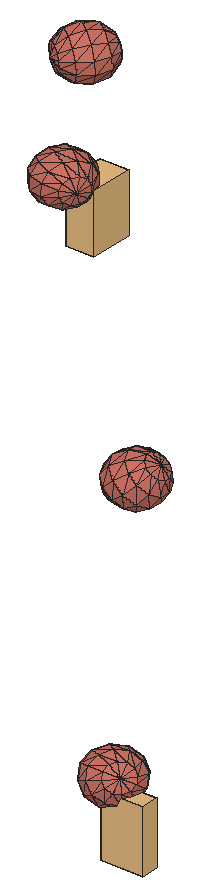
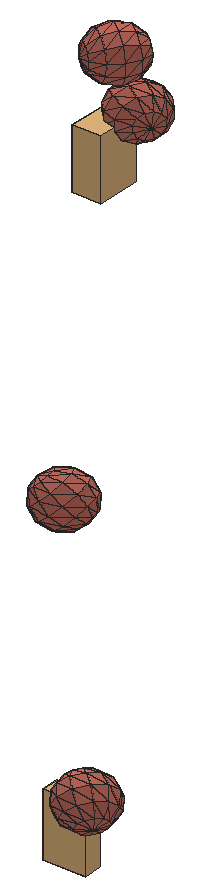
# SketchUp Ruby script. Lengths in inches.
U = 1.inch
M = Sketchup.active_model
def pt(a) = Geom::Point3d.new(a.map { |v| v * U })
def face(e, loops, mat)
  f = e.add_face(loops[0].map { |a| pt(a) })
  loops[1..].each { |l| e.add_face(l.map { |a| pt(a) }).erase! }
  f.material = f.back_material = mat if mat
  f
end
# faces: each face lists its corners as indices into pts; further lists are holes
def faces(e, pts, list, mat = nil) = list.each { |f| face(e, (f[0].is_a?(Array) ? f : [f]).map { |l| l.map { |i| pts[i] } }, mat) }
# xy, xz, yz: faces in a plane at the given z, y or x. An outline is a flat list of corners, or four numbers for a rectangle; further outlines are holes
def ring(l) = l.size == 4 ? [[l[0], l[1]], [l[2], l[1]], [l[2], l[3]], [l[0], l[3]]] : l.each_slice(2).to_a
def flat(e, list, mat, &to3) = list.each { |f| face(e, (f[0].is_a?(Array) ? f : [f]).map { |l| ring(l).map { |u, v| to3.(u, v) } }, mat) }
def xy(e, z, list, mat = nil) = flat(e, list, mat) { |x, y| [x, y, z] }
def xz(e, y, list, mat = nil) = flat(e, list, mat) { |x, z| [x, y, z] }
def yz(e, x, list, mat = nil) = flat(e, list, mat) { |y, z| [x, y, z] }
def lines(e, pts, list) = list.each { |a, b| e.add_line(pt(pts[a]), pt(pts[b])) }
# prism: a flat outline (further loops are holes) pulled along v
def prism(e, loops, v, mat = nil)
  f = face(e, loops, mat); d = Geom::Vector3d.new(v.map { |x| x * U })
  f.pushpull(f.normal.samedirection?(d) ? d.length : -d.length)
end
def box(e, o, s, mat = nil) = prism(e, [[o, [o[0] + s[0], o[1], o[2]], [o[0] + s[0], o[1] + s[1], o[2]], [o[0], o[1] + s[1], o[2]]]], [0, 0, s[2]], mat)
def at(x, y, z, deg = 0) = Geom::Transformation.translation(pt([x, y, z])) * Geom::Transformation.rotation(ORIGIN, Z_AXIS, deg.degrees)
def axes(o, x, y, z) = Geom::Transformation.new([*x, 0, *y, 0, *z, 0, *pt(o).to_a, 1])
def part(name) = M.definitions.add(name)
# library, detail: a bought-in or finely detailed component or shape, given as its bounding box
def library(name, o, s) = part(name).tap { |d| box(d.entities, o, s) }
def detail(e, o, s) = box(e.add_group.entities, o, s)
def put(e, d, t, mat = nil) = e.add_instance(d, t).tap { |i| i.material = mat if mat }
def group(e, t, mat = nil) = e.add_group.tap { |g| g.transformation = t; g.material = mat if mat }.entities
root = M.entities
M.materials.add("green").color = [174, 139, 102]
M.materials.add("vio").color = [206, 114, 100]
c1 = part("3DGeom~208_Defintion")
p = [[-278.9,104.85,-403.93],[-34.22,85.5625,-494.84],[-36.78,-106.97,-488.84],[218.15,-67.8125,-449.7],[219.62,43.35,-453.16],[33.05,253.77,-407.11],
  [-201.22,299.08,-302.625],[-278.9,104.85,-403.93],[-201.22,299.08,-302.625],[-281.85,-117.47,-397],[26.0625,-272.25,-390.72],[254.43,-163.24,-393.05],
  [-278.9,104.85,-403.93],[-281.85,-117.47,-397],[414.62,-10.48,-290.0625],[258.46,140.46,-402.51],[147.02,352.57,-249.16],[-69.62,413.17,-120.23],
  [33.05,253.77,-407.11],[-201.22,299.08,-302.625],[147.02,352.57,-249.16],[33.05,253.77,-407.11],[-448.85,96.04,-204.78],[-278.9,104.85,-403.93],
  [-281.85,-117.47,-397],[-381.57,264.25,-117.05],[-201.22,299.08,-302.625],[258.46,140.46,-402.51],[324.26,197.5,-311.32],[414.62,-10.48,-290.0625],
  [147.02,352.57,-249.16],[324.26,197.5,-311.32],[-451.4,-96.49,-198.78],[-209.29,-308.32,-283.69],[-281.85,-117.47,-397],[-209.29,-308.32,-283.69],
  [318.75,-217.36,-298.39],[318.75,-217.36,-298.39],[254.43,-163.24,-393.05],[414.62,-10.48,-290.0625],[-209.29,-308.32,-283.69],[26.0625,-272.25,-390.72],
  [137.48,-365.99,-226.76],[318.75,-217.36,-298.39],[137.48,-365.99,-226.76],[324.26,197.5,-311.32],[399.39,199.2,-204.01],[414.62,-10.48,-290.0625],
  [277.14,355.5,-63.3],[324.26,197.5,-311.32],[399.39,199.2,-204.01],[324.26,197.5,-311.32],[-267.6,363.06,40.9],[-201.22,299.08,-302.625],
  [-381.57,264.25,-117.05],[-267.6,363.06,40.9],[-201.22,299.08,-302.625],[318.75,-217.36,-298.39],[393.88,-215.66,-191.08],[393.88,-215.66,-191.08],
  [318.75,-217.36,-298.39],[414.62,-10.48,-290.0625],[459.68,-158.62,-99.89],[414.62,-10.48,-290.0625],[498.52,-61.5,-49.24],[414.62,-10.48,-290.0625],
  [500,49.66,-52.7],[414.62,-10.48,-290.0625],[399.39,199.2,-204.01],[463.72,145.08,-109.35],[414.62,-10.48,-290.0625],[414.62,-10.48,-290.0625],
  [-388.56,-261.77,-100.65],[-209.29,-308.32,-283.69],[-80.64,-416.55,-94.37],[-209.29,-308.32,-283.69],[-388.56,-261.77,-100.65],[80.64,416.55,94.37],
  [267.6,-363.06,-40.9],[393.88,-215.66,-191.08],[-498.52,61.5,49.24],[-459.68,158.62,99.89],[388.56,261.77,100.65],[399.39,199.2,-204.01],
  [388.56,261.77,100.65],[399.39,199.2,-204.01],[277.14,355.5,-63.3],[-500,-49.66,52.7],[267.6,-363.06,-40.9],[-137.48,365.99,226.76],
  [-267.6,363.06,40.9],[-393.88,215.66,191.08],[-267.6,363.06,40.9],[451.4,96.49,198.78],[388.56,261.77,100.65],[-388.56,-261.77,-100.65],
  [-277.14,-355.5,63.3],[-463.72,-145.08,109.35],[-277.14,-355.5,63.3],[267.6,-363.06,-40.9],[381.57,-264.25,117.05],[69.62,-413.17,120.23],
  [209.29,308.32,283.69],[388.56,261.77,100.65],[448.85,-96.04,204.78],[381.57,-264.25,117.05],[-318.75,217.36,298.39],[-267.6,363.06,40.9],
  [-393.88,215.66,191.08],[-318.75,217.36,298.39],[-267.6,363.06,40.9],[-414.62,10.48,290.0625],[-147.02,-352.57,249.16],[-277.14,-355.5,63.3],
  [-399.39,-199.2,204.01],[-399.39,-199.2,204.01],[-147.02,-352.57,249.16],[-26.0625,272.25,390.72],[-26.0625,272.25,390.72],[281.85,117.47,397],
  [388.56,261.77,100.65],[281.85,117.47,397],[388.56,261.77,100.65],[209.29,308.32,283.69],[381.57,-264.25,117.05],[201.22,-299.08,302.625],
  [201.22,-299.08,302.625],[-147.02,-352.57,249.16],[201.22,-299.08,302.625],[-318.75,217.36,298.39],[278.9,-104.85,403.93],[278.9,-104.85,403.93],
  [281.85,117.47,397],[-399.39,-199.2,204.01],[-147.02,-352.57,249.16],[-324.26,-197.5,311.32],[-324.26,-197.5,311.32],[201.22,-299.08,302.625],
  [278.9,-104.85,403.93],[-254.43,163.24,393.05],[-137.48,365.99,226.76],[-318.75,217.36,298.39],[-254.43,163.24,393.05],[-26.0625,272.25,390.72],
  [-137.48,365.99,226.76],[-324.26,-197.5,311.32],[-147.02,-352.57,249.16],[-33.05,-253.77,407.11],[-147.02,-352.57,249.16],[201.22,-299.08,302.625],
  [-33.05,-253.77,407.11],[36.78,106.98,488.84],[209.29,308.32,283.69],[281.85,117.47,397],[209.29,308.32,283.69],[-258.46,-140.46,402.51],
  [-258.46,-140.46,402.51],[-219.62,-43.35,453.16],[-414.62,10.48,290.0625],[-218.15,67.8125,449.7],[-414.62,10.48,290.0625],[-254.43,163.24,393.05],
  [-254.43,163.24,393.05],[-414.62,10.48,290.0625],[201.22,-299.08,302.625],[278.9,-104.85,403.93],[-324.26,-197.5,311.32],[-254.43,163.24,393.05],
  [34.22,-85.5625,494.84]]
faces(c1.entities,p,[[0,1,2],[1,3,2],[1,4,3],[5,4,1],[6,1,7],[8,5,1],[9,2,10],[2,11,10],
  [2,3,11],[12,2,13],[3,4,14],[4,15,14],[5,15,4],[11,3,14],[16,15,5],[17,18,19],
  [17,20,21],[22,23,24],[25,23,22],[25,26,23],[27,28,29],[30,31,15],[32,24,33],[34,10,35],
  [22,24,32],[10,11,36],[37,38,39],[40,41,42],[10,43,44],[45,46,47],[48,49,20],[48,50,51],
  [52,53,54],[55,17,56],[42,57,58],[59,60,61],[62,59,63],[64,62,65],[66,64,67],[68,69,70],
  [69,66,71],[72,73,74],[75,42,74],[32,33,76],[77,20,17],[77,48,20],[74,42,78],[42,79,78],
  [80,22,32],[81,22,80],[81,25,22],[82,69,83],[84,85,86],[87,32,76],[80,32,87],[88,59,62],
  [89,17,90],[89,77,17],[91,25,81],[91,92,25],[93,66,69],[93,69,94],[95,74,96],[97,76,98],
  [87,76,97],[99,62,100],[100,62,64],[96,74,101],[74,78,101],[102,103,48],[102,48,77],[104,64,66],
  [104,66,93],[100,64,104],[101,78,105],[106,107,108],[109,89,110],[80,87,111],[81,80,111],[87,97,111],
  [96,101,112],[97,113,114],[115,96,116],[117,77,89],[118,102,77],[91,81,111],[119,93,120],[121,122,123],
  [97,114,111],[101,124,125],[126,100,104],[127,101,128],[129,91,111],[130,104,93],[131,93,132],[133,134,135],
  [114,136,111],[137,104,138],[139,140,141],[142,143,144],[145,146,147],[148,149,150],[151,152,143],[151,153,154],
  [136,155,111],[156,157,158],[157,159,160],[161,129,111],[159,162,163],[147,164,165],[166,147,156],[159,143,167],
  [159,151,143],[168,165,153],[168,153,151],[156,147,168],[156,168,157],[147,165,168],[157,151,159],[157,168,151]],"vio")
c2 = part("3DGeom~244_Defintion")
p = [[-108.99,-83.02,-483.7],[90.05,60.9,-492.09],[201.25,-102.35,-447.625],[393.37,0,-317.28],[-208.69,-14.03,-459.98],[-82.63,180.41,-451.01],
  [264.97,188.51,-368.625],[-44.79,-177.28,-458.03],[-278.83,-204.71,-345.7],[-317.18,11.23,-393.23],[-33.3,-271.53,-389.85],[221.17,-265.61,-329.54],
  [221.17,-265.61,-329.54],[-270.53,224.16,-335.4],[65.57,326.51,-321.2],[416.36,-188.51,-180.93],[221.17,-265.61,-329.54],[416.36,-188.51,-180.93],
  [-405.375,-14.03,-301.34],[-405.375,-14.03,-301.34],[-270.53,224.16,-335.4],[-317.18,11.23,-393.23],[-33.3,-271.53,-389.85],[144.46,-385.12,-169.46],
  [-77.58,-340.53,-297.43],[-33.3,-271.53,-389.85],[221.17,-265.61,-329.54],[-77.58,-340.53,-297.43],[264.97,188.51,-368.625],[480.09,102.35,-101.93],
  [393.37,0,-317.28],[264.97,188.51,-368.625],[368.89,265.61,-146.39],[65.57,326.51,-321.2],[368.89,265.61,-146.39],[264.97,188.51,-368.625],
  [-165.78,-365.79,-205.53],[-165.78,-365.79,-205.53],[-274.26,-340.53,-138.79],[-278.83,-204.71,-345.7],[-274.26,-340.53,-138.79],[-373.96,-271.53,-115.07],
  [-278.83,-204.71,-345.7],[-438.16,-177.28,-140.74],[-278.83,-204.71,-345.7],[-449.66,-83.02,-208.92],[-405.375,-14.03,-301.34],[-278.83,-204.71,-345.7],
  [-278.83,-204.71,-345.7],[-405.375,-14.03,-301.34],[-423.3,180.41,-176.24],[-270.53,224.16,-335.4],[-151.39,377.02,-187.7],[-270.53,224.16,-335.4],
  [-151.39,377.02,-187.7],[327.8,-326.51,3.91],[416.36,-188.51,-180.93],[65.57,326.51,-321.2],[196.2,385.12,-105.3125],[368.89,265.61,-146.39],
  [-151.39,377.02,-187.7],[65.57,326.51,-321.2],[393.37,0,-317.28],[500,-60.9,16.16],[416.36,-188.51,-180.93],[393.37,0,-317.28],
  [-405.375,-14.03,-301.34],[-77.58,-340.53,-297.43],[-8.31,-428.86,-10.3],[-165.78,-365.79,-205.53],[-77.58,-340.53,-297.43],[-500,60.9,-16.16],
  [-165.78,-365.79,-205.53],[-196.2,-385.12,105.3125],[-165.78,-365.79,-205.53],[-274.26,-340.53,-138.79],[-327.8,326.51,-3.91],[-151.39,377.02,-187.7],
  [-327.8,326.51,-3.91],[8.31,428.86,10.3],[-151.39,377.02,-187.7],[-151.39,377.02,-187.7],[416.36,-188.51,-180.93],[423.3,-180.41,176.24],
  [327.8,-326.51,3.91],[416.36,-188.51,-180.93],[151.39,-377.02,187.7],[438.16,177.28,140.74],[373.96,271.53,115.07],[373.96,271.53,115.07],
  [368.89,265.61,-146.39],[-480.09,-102.35,101.93],[-274.26,-340.53,-138.79],[-368.89,-265.61,146.39],[-274.26,-340.53,-138.79],[-368.89,-265.61,146.39],
  [-373.96,-271.53,-115.07],[-368.89,-265.61,146.39],[274.26,340.53,138.79],[373.96,271.53,115.07],[449.66,83.02,208.92],[-416.36,188.51,180.93],
  [-65.57,-326.51,321.2],[-416.36,188.51,180.93],[-144.46,385.12,169.46],[-327.8,326.51,-3.91],[-327.8,326.51,-3.91],[327.8,-326.51,3.91],
  [270.53,-224.16,335.4],[151.39,-377.02,187.7],[327.8,-326.51,3.91],[165.78,365.79,205.53],[405.375,14.03,301.34],[-393.37,0,317.28],
  [-264.97,-188.51,368.625],[-368.89,-265.61,146.39],[-264.97,-188.51,368.625],[278.83,204.71,345.7],[274.26,340.53,138.79],[278.83,204.71,345.7],
  [278.83,204.71,345.7],[278.83,204.71,345.7],[-264.97,-188.51,368.625],[-416.36,188.51,180.93],[-221.17,265.61,329.54],[77.58,340.54,297.43],
  [317.18,-11.23,393.23],[-393.37,0,317.28],[-221.17,265.61,329.54],[-416.36,188.51,180.93],[151.39,-377.02,187.7],[82.63,-180.41,451.01],
  [-65.57,-326.51,321.2],[151.39,-377.02,187.7],[270.53,-224.16,335.4],[165.78,365.79,205.53],[77.58,340.54,297.43],[278.83,204.71,345.7],
  [278.83,204.71,345.7],[77.58,340.54,297.43],[33.3,271.53,389.85],[33.3,271.53,389.85],[317.18,-11.23,393.23],[405.375,14.03,301.34],
  [-264.97,-188.51,368.625],[-201.25,102.35,447.625],[-393.37,0,317.28],[-393.37,0,317.28],[-221.17,265.61,329.54],[-65.57,-326.51,321.2],
  [-90.05,-60.9,492.09],[-264.97,-188.51,368.625],[-65.57,-326.51,321.2],[33.3,271.53,389.85],[-221.17,265.61,329.54],[270.53,-224.16,335.4],
  [208.69,14.03,459.98],[270.53,-224.16,335.4],[317.18,-11.23,393.23],[317.18,-11.23,393.23],[108.99,83.02,483.7],[44.79,177.28,458.03],
  [33.3,271.53,389.85],[-264.97,-188.51,368.625],[33.3,271.53,389.85]]
faces(c2.entities,p,[[0,1,2],[1,3,2],[4,1,0],[4,5,1],[1,6,3],[5,6,1],[0,7,8],[4,0,8],
  [0,2,7],[9,4,8],[9,5,4],[7,10,8],[7,11,10],[7,2,12],[9,13,5],[13,14,5],
  [5,14,6],[2,15,16],[2,3,17],[18,9,8],[19,20,21],[22,23,24],[25,26,23],[10,27,8],
  [28,29,30],[31,32,29],[33,34,35],[27,36,8],[37,38,39],[40,41,42],[41,43,44],[45,46,47],
  [43,45,48],[49,50,51],[50,52,53],[13,54,14],[26,55,23],[26,56,55],[57,58,59],[60,58,61],
  [62,63,64],[65,29,63],[45,50,66],[67,68,69],[70,23,68],[43,71,45],[45,71,50],[72,68,73],
  [74,73,75],[50,76,77],[78,79,80],[81,79,58],[82,83,84],[85,63,83],[71,76,50],[23,86,68],
  [23,55,86],[32,87,29],[32,88,87],[58,89,90],[41,91,43],[43,91,71],[92,73,93],[94,95,96],
  [41,97,91],[58,98,99],[79,98,58],[29,100,63],[29,87,100],[91,101,71],[71,101,76],[68,102,73],
  [68,86,102],[103,104,105],[106,104,79],[107,108,109],[110,83,108],[79,111,98],[104,111,79],[63,112,83],
  [63,100,112],[97,113,91],[91,113,101],[73,114,115],[73,102,116],[87,88,117],[88,118,119],[98,111,120],
  [100,87,121],[97,122,113],[123,124,104],[124,125,104],[104,125,111],[83,126,108],[83,112,126],[127,128,129],
  [130,131,132],[133,134,131],[135,136,137],[112,100,138],[139,140,137],[124,141,125],[142,143,137],[144,145,146],
  [147,145,148],[149,150,151],[152,131,150],[145,153,154],[155,156,131],[157,158,156],[156,159,137],[160,156,137],
  [161,160,137],[162,161,137],[163,150,145],[145,161,164],[150,161,145],[131,160,150],[131,156,160],[150,160,161]],"vio")
c3 = part("3DGeom~248_Defintion")
p = [[242.2,-95.53,-426.77],[-5.12,-61.18,-498.23],[-8.42,49.39,-500],[242.2,-95.53,-426.77],[236.48,95.97,-429.83],[-251.07,-10.43,-436.2],
  [-67.73,144.3,-469.01],[149.39,-262.83,-367.79],[-58.71,-157.77,-464.19],[242.2,-95.53,-426.77],[-167.15,198.125,-413.57],[133.76,260.36,-376.15],
  [133.76,260.36,-376.15],[-17.09,-361.11,-268.71],[-154.82,-214.51,-406.98],[-17.09,-361.11,-268.71],[-267.71,-216.1875,-341.94],[-367.14,-162.36,-286.51],
  [-267.71,-216.1875,-341.94],[-367.14,-162.36,-286.51],[-426.44,-67.45,-255.52],[-426.44,-67.45,-255.52],[-429.75,43.11,-257.28],[-251.07,-10.43,-436.2],
  [-429.75,43.11,-257.28],[-376.16,139.71,-291.33],[-376.16,139.71,-291.33],[-280.04,196.44,-348.54],[-280.04,196.44,-348.54],[424.625,-104.29,-240.95],
  [242.2,-95.53,-426.77],[236.48,95.97,-429.83],[236.48,95.97,-429.83],[418.02,116.84,-244.48],[418.02,116.84,-244.48],[133.76,260.36,-376.15],
  [317.45,-297.47,-172.85],[242.2,-95.53,-426.77],[317.45,-297.47,-172.85],[242.2,-95.53,-426.77],[424.625,-104.29,-240.95],[-38.44,353.59,-280.13],
  [-280.04,196.44,-348.54],[133.76,260.36,-376.15],[-38.44,353.59,-280.13],[-212.625,-364.02,-156.07],[-267.71,-216.1875,-341.94],[-154.82,-214.51,-406.98],
  [-154.82,-214.51,-406.98],[-17.09,-361.11,-268.71],[418.02,116.84,-244.48],[133.76,260.36,-376.15],[299.4,306.66,-182.51],[299.4,306.66,-182.51],
  [133.76,260.36,-376.15],[-38.44,353.59,-280.13],[125.22,-410.95,-58.44],[149.39,-262.83,-367.79],[149.39,-262.83,-367.79],[317.45,-297.47,-172.85],
  [-233.98,350.68,-167.49],[-280.04,196.44,-348.54],[-376.16,139.71,-291.33],[-38.44,353.59,-280.13],[-280.04,196.44,-348.54],[-233.98,350.68,-167.49],
  [-384.83,-270.79,-60.04],[-267.71,-216.1875,-341.94],[-212.625,-364.02,-156.07],[-367.14,-162.36,-286.51],[-267.71,-216.1875,-341.94],[-400.46,252.4,-68.4],
  [-233.98,350.68,-167.49],[-487.55,-106.4,-6.37],[100.5625,414.3125,-71.63],[-233.98,350.68,-167.49],[-100.5625,-414.3125,71.63],[-493.27,85.1,-9.43],
  [493.27,-85.1,9.43],[487.55,106.4,6.37],[299.4,306.66,-182.51],[400.46,-252.4,68.4],[317.45,-297.47,-172.85],[299.4,306.66,-182.51],
  [384.83,270.79,60.04],[384.83,270.79,60.04],[233.98,-350.68,167.49],[317.45,-297.47,-172.85],[233.98,-350.68,167.49],[317.45,-297.47,-172.85],
  [400.46,-252.4,68.4],[-125.22,410.95,58.44],[-400.46,252.4,-68.4],[-299.4,-306.66,182.51],[-299.4,-306.66,182.51],[-384.83,-270.79,-60.04],
  [384.83,270.79,60.04],[212.625,364.02,156.07],[-317.45,297.47,172.85],[-400.46,252.4,-68.4],[-317.45,297.47,172.85],[-418.02,-116.84,244.48],
  [-299.4,-306.66,182.51],[-418.02,-116.84,244.48],[38.44,-353.59,280.13],[38.44,-353.59,280.13],[233.98,-350.68,167.49],[-424.625,104.29,240.95],
  [-317.45,297.47,172.85],[-418.02,-116.84,244.48],[429.75,-43.11,257.28],[426.44,67.45,255.52],[426.44,67.45,255.52],[376.16,-139.71,291.33],
  [376.16,-139.71,291.33],[17.09,361.11,268.71],[-317.45,297.47,172.85],[17.09,361.11,268.71],[426.44,67.45,255.52],[367.14,162.36,286.51],
  [367.14,162.36,286.51],[212.625,364.02,156.07],[280.04,-196.44,348.54],[233.98,-350.68,167.49],[280.04,-196.44,348.54],[376.16,-139.71,291.33],
  [-133.76,-260.36,376.15],[-299.4,-306.66,182.51],[-133.76,-260.36,376.15],[38.44,-353.59,280.13],[367.14,162.36,286.51],[212.625,364.02,156.07],
  [267.71,216.1875,341.94],[267.71,216.1875,341.94],[17.09,361.11,268.71],[167.15,-198.125,413.57],[38.44,-353.59,280.13],[233.98,-350.68,167.49],
  [233.98,-350.68,167.49],[280.04,-196.44,348.54],[-149.39,262.83,367.79],[-317.45,297.47,172.85],[-424.625,104.29,240.95],[17.09,361.11,268.71],
  [-317.45,297.47,172.85],[-149.39,262.83,367.79],[-236.48,-95.97,429.83],[-418.02,-116.84,244.48],[-299.4,-306.66,182.51],[-133.76,-260.36,376.15],
  [-242.2,95.53,426.77],[-418.02,-116.84,244.48],[-424.625,104.29,240.95],[-242.2,95.53,426.77],[-242.2,95.53,426.77],[-418.02,-116.84,244.48],
  [-236.48,-95.97,429.83],[426.44,67.45,255.52],[251.07,10.43,436.2],[426.44,67.45,255.52],[367.14,162.36,286.51],[251.07,10.43,436.2],
  [376.16,-139.71,291.33],[429.75,-43.11,257.28],[154.82,214.51,406.98],[17.09,361.11,268.71],[267.71,216.1875,341.94],[17.09,361.11,268.71],
  [154.82,214.51,406.98],[67.73,-144.3,469.01],[267.71,216.1875,341.94],[58.71,157.77,464.19],[8.42,-49.39,500],[5.12,61.18,498.23]]
faces(c3.entities,p,[[0,1,2],[3,2,4],[2,1,5],[6,2,5],[4,2,6],[7,8,1],[7,1,9],[1,8,5],
  [10,6,5],[4,6,11],[12,6,10],[13,14,8],[15,8,7],[8,14,5],[16,17,5],[14,18,5],
  [19,20,5],[21,22,23],[24,25,5],[26,27,5],[28,10,5],[29,30,31],[29,32,33],[34,4,35],
  [36,7,37],[38,39,40],[41,10,42],[43,10,44],[45,46,47],[45,48,49],[50,51,52],[53,54,55],
  [56,49,57],[56,58,59],[60,61,62],[63,64,65],[66,67,68],[66,69,70],[71,62,22],[72,62,71],
  [73,69,66],[73,21,69],[53,55,74],[74,55,75],[76,45,49],[76,49,56],[77,22,21],[71,22,77],
  [77,21,73],[78,29,33],[78,33,79],[79,33,80],[81,82,29],[81,29,78],[79,83,84],[85,53,74],
  [86,56,87],[88,89,90],[91,75,92],[74,75,91],[93,45,76],[94,95,45],[96,74,97],[97,74,91],
  [98,71,77],[91,99,100],[101,66,102],[103,73,66],[104,76,56],[105,56,106],[107,77,73],[108,77,107],
  [107,73,109],[110,78,79],[110,79,111],[112,79,84],[113,81,78],[114,78,110],[115,91,116],[97,91,117],
  [118,84,119],[120,84,121],[122,123,81],[124,81,125],[126,127,76],[128,76,129],[130,131,132],[133,97,134],
  [135,136,137],[135,138,139],[140,141,142],[143,144,145],[146,147,148],[146,148,149],[150,107,151],[140,152,153],
  [154,155,156],[110,157,158],[159,160,161],[162,163,161],[164,165,140],[166,167,168],[169,149,136],[169,136,135],
  [160,170,161],[139,162,161],[170,164,161],[135,139,161],[171,140,153],[164,140,171],[172,146,149],[172,149,169],
  [164,171,161],[169,135,161],[173,153,146],[171,153,173],[173,146,172],[172,169,161],[173,172,161],[171,173,161]],"vio")
c4 = part("3DGeom~241_Defintion")
p = [[-83.63,87.77,-500],[-95.35,-182.17,-461.02],[-273.19,-13.21,-439.1],[14.09,-123.87,-496.18],[142.8125,124.74,-475.08],[-158.95,275.9,-369.85],
  [-273.19,-13.21,-439.1],[102.53,318.58,-341.07],[-158.95,275.9,-369.85],[102.53,318.58,-341.07],[108.04,-302.32,-359.41],[144.83,-102.53,-481.79],
  [108.04,-302.32,-359.41],[261.83,-123.87,-421.71],[108.04,-302.32,-359.41],[345.47,87.77,-371.01],[336.53,275.9,-220.9],[336.53,275.9,-220.9],
  [102.53,318.58,-341.07],[-154.17,-261.82,-385.73],[108.04,-302.32,-359.41],[-273.19,-13.21,-439.1],[-273.19,-13.21,-439.1],[-375.08,-151.16,-308.7],
  [-377.83,159.29,-299.52],[-273.19,-13.21,-439.1],[-375.08,-151.16,-308.7],[-158.95,275.9,-369.85],[-273.19,-13.21,-439.1],[-377.83,159.29,-299.52],
  [333.75,-182.17,-332.03],[108.04,-302.32,-359.41],[470.03,-13.21,-215.68],[333.75,-182.17,-332.03],[261.83,-123.87,-421.71],[261.83,-123.87,-421.71],
  [345.47,87.77,-371.01],[-375.08,-151.16,-308.7],[-146.61,-341.47,-290.49],[-146.61,-341.47,-290.49],[108.04,-302.32,-359.41],[480.36,159.29,-41.54],
  [345.47,87.77,-371.01],[345.47,87.77,-371.01],[336.53,275.9,-220.9],[-191.67,390.1,-140.59],[-158.95,275.9,-369.85],[34.77,427.0625,-115.67],
  [-158.95,275.9,-369.85],[-191.67,390.1,-140.59],[102.53,318.58,-341.07],[-158.95,275.9,-369.85],[42.3,-421.11,-140.72],[-74.7,-399.77,-200.81],
  [108.04,-302.32,-359.41],[173.04,-399.77,-126.33],[-146.61,-341.47,-290.49],[282.49,-341.47,-161.49],[341.31,-261.82,-236.78],[282.49,-341.47,-161.49],
  [333.75,-182.17,-332.03],[341.31,-261.82,-236.78],[108.04,-302.32,-359.41],[237.42,390.1,-11.6],[336.53,275.9,-220.9],[483.12,-151.16,-50.71],
  [341.31,-261.82,-236.78],[-375.08,-151.16,-308.7],[-146.61,-341.47,-290.49],[-361.98,-289.11,-143.73],[-495.48,0,-148.95],[-361.98,-289.11,-143.73],
  [-381.24,289.11,-79.69],[-191.67,390.1,-140.59],[-361.98,-289.11,-143.73],[381.24,-289.11,79.69],[282.49,-341.47,-161.49],[361.98,289.11,143.73],
  [336.53,275.9,-220.9],[361.98,289.11,143.73],[336.53,275.9,-220.9],[237.42,390.1,-11.6],[495.48,0,148.95],[-237.42,-390.1,11.6],
  [-361.98,-289.11,-143.73],[191.67,-390.1,140.59],[282.49,-341.47,-161.49],[191.67,-390.1,140.59],[282.49,-341.47,-161.49],[381.24,-289.11,79.69],
  [-480.36,-159.29,41.54],[-483.12,151.16,50.71],[-237.42,-390.1,11.6],[-34.77,-427.0625,115.67],[-173.04,399.77,126.33],[-381.24,289.11,-79.69],
  [-42.3,421.11,140.72],[191.67,-390.1,140.59],[74.7,399.77,200.81],[-282.49,341.47,161.5],[-381.24,289.11,-79.69],[-282.49,341.47,161.5],
  [377.83,-159.29,299.53],[375.08,151.16,308.7],[375.08,151.16,308.7],[361.98,289.11,143.73],[146.61,341.47,290.49],[361.98,289.11,143.73],
  [-336.53,-275.9,220.9],[-237.42,-390.1,11.6],[-336.53,-275.9,220.9],[-470.03,13.21,215.68],[-336.53,-275.9,220.9],[-341.31,261.82,236.78],
  [-282.49,341.47,161.5],[-341.31,261.82,236.78],[158.95,-275.9,369.85],[191.67,-390.1,140.59],[158.95,-275.9,369.85],[-336.53,-275.9,220.9],
  [-102.53,-318.58,341.07],[-102.53,-318.58,341.07],[191.67,-390.1,140.59],[-108.04,302.32,359.41],[-108.04,302.32,359.41],[-102.53,-318.58,341.07],
  [191.67,-390.1,140.59],[158.95,-275.9,369.85],[-108.04,302.32,359.41],[154.17,261.82,385.73],[375.08,151.16,308.7],[361.98,289.11,143.73],
  [361.98,289.11,143.73],[146.61,341.47,290.49],[273.19,13.21,439.1],[273.19,13.21,439.1],[375.08,151.16,308.7],[-341.31,261.82,236.78],
  [-108.04,302.32,359.41],[-108.04,302.32,359.41],[-336.53,-275.9,220.9],[-345.47,-87.77,371.01],[-333.75,182.17,332.03],[-345.47,-87.77,371.01],
  [-341.31,261.82,236.78],[-333.75,182.17,332.03],[-345.47,-87.77,371.01],[-336.53,-275.9,220.9],[-102.53,-318.58,341.07],[-341.31,261.82,236.78],
  [-333.75,182.17,332.03],[-108.04,302.32,359.41],[146.61,341.47,290.49],[83.63,-87.77,500],[158.95,-275.9,369.85],[377.83,-159.29,299.53],
  [377.83,-159.29,299.53],[273.19,13.21,439.1],[95.35,182.17,461.02],[-333.75,182.17,332.03],[-345.47,-87.77,371.01],[-261.83,123.87,421.71],
  [-261.83,123.87,421.71],[-142.8125,-124.74,475.08],[-144.83,102.53,481.79],[-14.09,123.87,496.18]]
faces(c4.entities,p,[[0,1,2],[0,3,1],[4,3,0],[5,0,6],[7,0,8],[9,4,0],[1,3,10],[3,11,12],
  [4,11,3],[11,13,14],[15,13,11],[15,11,4],[16,15,4],[17,4,18],[19,1,20],[21,1,19],
  [22,19,23],[24,25,26],[27,28,29],[13,30,31],[32,33,34],[32,35,36],[37,19,38],[39,19,40],
  [41,32,42],[41,43,44],[45,46,24],[47,48,49],[47,50,51],[52,53,54],[55,52,54],[53,56,54],
  [57,55,54],[58,59,54],[60,61,62],[63,64,50],[63,50,47],[65,66,33],[65,33,32],[67,68,69],
  [70,26,71],[24,26,70],[72,24,70],[73,24,72],[74,56,53],[75,76,66],[75,66,65],[77,41,78],
  [79,80,81],[82,65,32],[82,32,41],[83,53,52],[84,53,83],[85,55,86],[87,88,89],[70,71,90],
  [91,70,90],[72,70,91],[90,71,92],[83,52,93],[93,52,55],[94,49,95],[96,47,49],[96,49,94],
  [93,55,97],[98,63,47],[98,47,96],[99,72,91],[94,100,101],[102,75,65],[102,65,82],[103,82,41],
  [104,41,105],[106,107,63],[106,63,98],[108,83,93],[90,109,110],[111,90,112],[91,90,111],[113,91,111],
  [114,91,115],[116,117,75],[118,75,102],[119,93,120],[121,93,122],[94,101,123],[96,94,124],[125,126,127],
  [98,96,128],[129,130,131],[129,132,133],[134,102,82],[135,82,136],[101,137,138],[106,98,139],[111,140,141],
  [142,111,143],[144,111,145],[146,147,148],[149,150,151],[129,152,151],[153,154,155],[153,156,157],[158,157,130],
  [158,130,129],[159,160,161],[150,162,151],[146,148,163],[163,148,154],[162,164,151],[164,165,151],[165,158,151],
  [158,129,151],[163,154,153],[162,146,163],[162,163,164],[165,153,157],[165,157,158],[164,163,153],[164,153,165]],"vio")
c5 = library("3DGeom~173_Defintion",[-146.02,-500,-341.01],[292.04,1000,682.02])
c6 = part("3DGeom~174_Defintion")
p = [[-127.07,494.74,-302.98],[-83.38,461.51,-336.48],[-100.9,461.46,-341.01],[-127.07,494.74,-302.98],[-117.78,466.57,-338.44],[-127.07,494.74,-302.98],
  [-117.78,466.57,-338.44],[-129.48,475.47,-329.47],[-127.07,494.74,-302.98],[-69.91,466.72,-326.0625],[-127.07,494.74,-302.98],[-129.48,475.47,-329.47],
  [-132.89,485.78,-316.49],[-127.07,494.74,-302.98],[-64.09,475.68,-312.56],[-69.91,466.72,-326.0625],[-127.07,494.74,-302.98],[-67.49,485.99,-299.58],
  [-64.09,475.68,-312.56],[-127.07,494.74,-302.98],[-79.2,494.89,-290.61],[-67.49,485.99,-299.58],[-127.07,494.74,-302.98],[-113.59,499.94,-292.57],
  [-96.07,500,-288.04],[-127.07,494.74,-302.98],[-96.07,500,-288.04],[-79.2,494.89,-290.61],[109.52,-498.77,278.33],[81.81,-497.43,299.58],
  [93.08,-500,285.75],[109.52,-498.77,278.33],[84.66,-484.5,330.92],[81.81,-497.43,299.58],[140.09,-487.18,288.41],[84.66,-484.5,330.92],
  [109.52,-498.77,278.33],[140.09,-487.18,288.41],[109.52,-498.77,278.33],[126.73,-494.08,279.3],[142.9375,-474.24,319.75],[84.66,-484.5,330.92],
  [140.09,-487.18,288.41],[142.9375,-474.24,319.75],[140.09,-487.18,288.41],[146.02,-479.92,303.22],[84.66,-484.5,330.92],[78.73,-491.76,316.12],
  [81.81,-497.43,299.58],[115.22,-472.9,341.01],[84.66,-484.5,330.92],[142.9375,-474.24,319.75],[115.22,-472.9,341.01],[142.9375,-474.24,319.75],
  [131.66,-471.68,333.58],[84.66,-484.5,330.92],[115.22,-472.9,341.01],[98.02,-477.6,340.03]]
faces(c6.entities,p,[[0,1,2],[3,2,4],[5,6,7],[8,9,1],[10,11,12],[13,14,15],[16,17,18],[19,20,21],
  [22,23,24],[25,26,27],[28,29,30],[31,32,33],[34,35,36],[37,38,39],[40,41,42],[43,44,45],
  [46,47,48],[49,50,51],[52,53,54],[55,56,57]],"green")
c7 = library("3DGeom~181_Defintion",[-363.49,-500,-241.625],[726.98,1000,483.25])
c8 = part("3DGeom~182_Defintion")
p = [[358.51,487.39,-222.91],[326.92,489.88,-241.625],[308.78,492.93,-236.98],[358.51,487.39,-222.91],[345.12,487.85,-236.47],[326.92,489.88,-241.625],
  [358.51,487.39,-222.91],[308.78,492.93,-236.98],[295.57,496.1875,-223.79],[358.51,487.39,-222.91],[295.57,496.1875,-223.79],[290.82,498.77,-205.58],
  [358.51,487.39,-222.91],[290.82,498.77,-205.58],[295.8,500,-187.23],[358.51,487.39,-222.91],[295.8,500,-187.23],[309.18,499.54,-173.67],
  [358.51,487.39,-222.91],[309.18,499.54,-173.67],[327.38,497.51,-168.51],[358.51,487.39,-222.91],[327.38,497.51,-168.51],[345.52,494.46,-173.16],
  [358.51,487.39,-222.91],[345.52,494.46,-173.16],[358.74,491.2,-186.35],[358.51,487.39,-222.91],[358.74,491.2,-186.35],[363.49,488.61,-204.5625],
  [-336.99,-490.37,173.04],[-308.93,-500,194.02],[-361.3125,-469.79,186.35],[-308.93,-500,194.02],[-336.99,-490.37,173.04],[-321.37,-497.625,179.85],
  [-336.99,-490.37,173.04],[-361.3125,-469.79,186.35],[-351.61,-480.18,175.42],[-361.3125,-469.79,186.35],[-308.93,-500,194.02],[-357.5625,-458.84,220.65],
  [-361.3125,-469.79,186.35],[-357.5625,-458.84,220.65],[-363.49,-461.98,202.91],[-357.5625,-458.84,220.65],[-308.93,-500,194.02],[-329.5,-468.47,241.625],
  [-329.5,-468.47,241.625],[-308.93,-500,194.02],[-305.18,-489.05,228.31],[-308.93,-500,194.02],[-303,-496.86,211.76],[-305.18,-489.05,228.31],
  [-357.5625,-458.84,220.65],[-329.5,-468.47,241.625],[-345.12,-461.21,234.82],[-329.5,-468.47,241.625],[-305.18,-489.05,228.31],[-314.88,-478.66,239.24]]
faces(c8.entities,p,[[0,1,2],[3,4,5],[6,7,8],[9,10,11],[12,13,14],[15,16,17],[18,19,20],[21,22,23],
  [24,25,26],[27,28,29],[30,31,32],[33,34,35],[36,37,38],[39,40,41],[42,43,44],[45,46,47],
  [48,49,50],[51,52,53],[54,55,56],[57,58,59]],"green")
g1 = group(root,at(15.3125,134.49,26.21))
put(g1,c1,axes([-1.55,-0.47,14.8],[0,0.00039,0],[0,0,-0.00039],[-0.00039,0,0]),"vio")
g2 = group(root,at(15.3125,134.49,26.21))
put(g2,c2,axes([-1.47,-0.33,10.38],[0,0.00039,0],[0,0,-0.00039],[-0.00039,0,0]),"vio")
g3 = group(root,at(15.3125,134.49,26.21))
put(g3,c3,axes([-1.41,-0.83,14.25],[0,0.00039,0],[0,0,-0.00039],[-0.00039,0,0]),"vio")
g4 = group(root,at(15.3125,134.49,26.21))
put(g4,c4,axes([-1.38,-0.25,12.18],[0,0.00038,0],[0,0,-0.00038],[-0.00038,0,0]),"vio")
g5 = group(root,at(15.3125,134.49,26.21))
put(g5,c5,axes([-1.32,-0.39,10.14],[0,0.00042,0],[0,0,-0.00042],[-0.00042,0,0]),"green")
put(g5,c6,axes([-1.32,-0.39,10.14],[0,0.00042,0],[0,0,-0.00042],[-0.00042,0,0]),"green")
g6 = group(root,at(15.3125,134.49,26.21))
put(g6,c7,axes([-1.31,-0.67,14.03],[0,0.0004,0],[0,0,-0.0004],[-0.0004,0,0]),"green")
put(g6,c8,axes([-1.31,-0.67,14.03],[0,0.0004,0],[0,0,-0.0004],[-0.0004,0,0]),"green")
